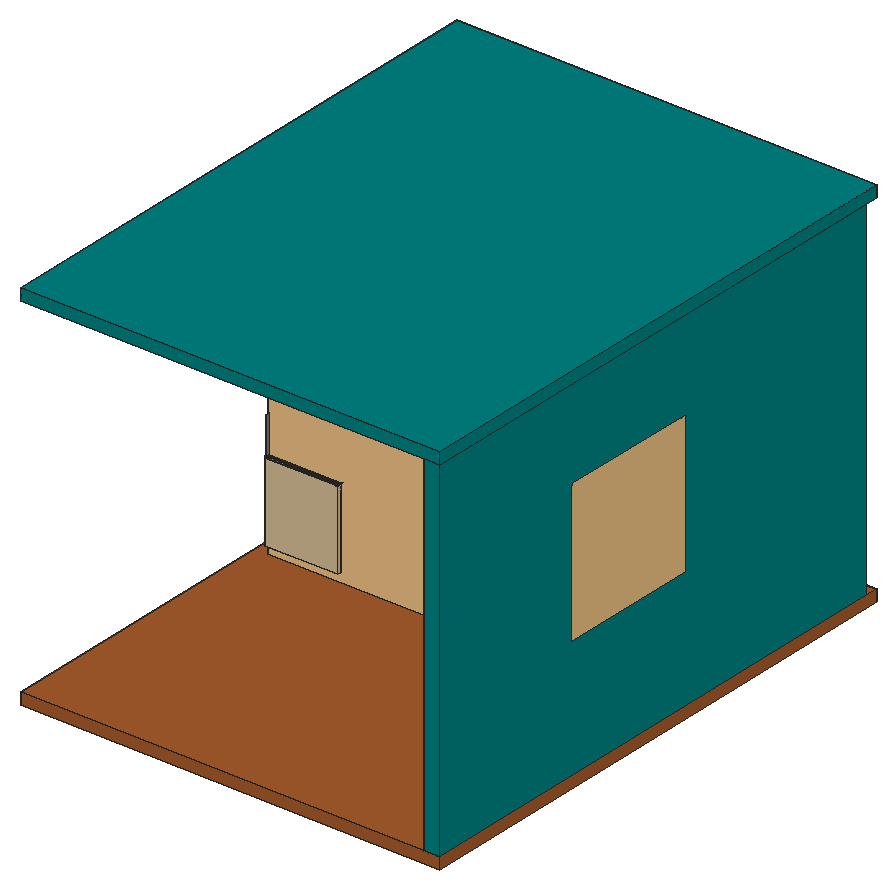
# SketchUp Ruby script. Lengths in inches.
U = 1.inch
M = Sketchup.active_model
def pt(a) = Geom::Point3d.new(a.map { |v| v * U })
def face(e, loops, mat)
  f = e.add_face(loops[0].map { |a| pt(a) })
  loops[1..].each { |l| e.add_face(l.map { |a| pt(a) }).erase! }
  f.material = f.back_material = mat if mat
  f
end
# faces: each face lists its corners as indices into pts; further lists are holes
def faces(e, pts, list, mat = nil) = list.each { |f| face(e, (f[0].is_a?(Array) ? f : [f]).map { |l| l.map { |i| pts[i] } }, mat) }
# xy, xz, yz: faces in a plane at the given z, y or x. An outline is a flat list of corners, or four numbers for a rectangle; further outlines are holes
def ring(l) = l.size == 4 ? [[l[0], l[1]], [l[2], l[1]], [l[2], l[3]], [l[0], l[3]]] : l.each_slice(2).to_a
def flat(e, list, mat, &to3) = list.each { |f| face(e, (f[0].is_a?(Array) ? f : [f]).map { |l| ring(l).map { |u, v| to3.(u, v) } }, mat) }
def xy(e, z, list, mat = nil) = flat(e, list, mat) { |x, y| [x, y, z] }
def xz(e, y, list, mat = nil) = flat(e, list, mat) { |x, z| [x, y, z] }
def yz(e, x, list, mat = nil) = flat(e, list, mat) { |y, z| [x, y, z] }
def lines(e, pts, list) = list.each { |a, b| e.add_line(pt(pts[a]), pt(pts[b])) }
# prism: a flat outline (further loops are holes) pulled along v
def prism(e, loops, v, mat = nil)
  f = face(e, loops, mat); d = Geom::Vector3d.new(v.map { |x| x * U })
  f.pushpull(f.normal.samedirection?(d) ? d.length : -d.length)
end
def box(e, o, s, mat = nil) = prism(e, [[o, [o[0] + s[0], o[1], o[2]], [o[0] + s[0], o[1] + s[1], o[2]], [o[0], o[1] + s[1], o[2]]]], [0, 0, s[2]], mat)
def at(x, y, z, deg = 0) = Geom::Transformation.translation(pt([x, y, z])) * Geom::Transformation.rotation(ORIGIN, Z_AXIS, deg.degrees)
def axes(o, x, y, z) = Geom::Transformation.new([*x, 0, *y, 0, *z, 0, *pt(o).to_a, 1])
def part(name) = M.definitions.add(name)
# library, detail: a bought-in or finely detailed component or shape, given as its bounding box
def library(name, o, s) = part(name).tap { |d| box(d.entities, o, s) }
def detail(e, o, s) = box(e.add_group.entities, o, s)
def put(e, d, t, mat = nil) = e.add_instance(d, t).tap { |i| i.material = mat if mat }
def group(e, t, mat = nil) = e.add_group.tap { |g| g.transformation = t; g.material = mat if mat }.entities
root = M.entities
M.materials.add("CLC2-PC-Blanc INTER").color = [249, 249, 249]
M.materials.add("Material \#1").color = [0, 0, 0]
M.materials.add("Standardmaterial30").color = [86, 86, 86]
M.materials.add("[0031_PapayaWhip]").color = [199, 195, 183]
M.materials.add("[0031_PapayaWhip]1").color = [211, 117, 3]
M.materials.add("[0079_Teal]").color = [0, 128, 128]
M.materials.add("[0091_MintCream]").color = [201, 113, 3]
M.materials.add("[0099_LightSteelBlue]").color = [176, 196, 222]
M.materials.add("[Blacktop Old 01]").color = [132, 136, 139]
M.materials.add("[Blinds Wood White]").color = [138, 137, 139]
M.materials.add("[Encaustic Tile Circular 01]").color = [123, 123, 122]
M.materials.add("[Formica Beige]").color = [211, 187, 149]
M.materials.add("[Ornate Tile 01]").color = [202, 202, 202]
M.materials.add("[Resin Turquoise]").color = [117, 218, 223]
M.materials.add("[Stone Marble]").color = [143, 138, 136]
M.materials.add("[Stone Vein Gray]").color = [166, 165, 165]
M.materials.add("[Terrazzo Light Blue]").color = [196, 214, 227]
M.materials.add("[Tile Hexagon White]").color = [213, 206, 204]
M.materials.add("[Translucent Glass Gray]").color = [128, 128, 128]
M.materials["[Translucent Glass Gray]"].alpha = 0.5
M.materials.add("[Wood Board Cork]").color = [215, 201, 115]
M.materials.add("[Wood Cherry Original]").color = [152, 86, 42]
M.materials.add("[Wood Square Tile 01]").color = [164, 91, 44]
M.materials.add("utensils_wood_2").color = [89, 58, 24]
c1 = library("Group\#12",[-32.31,-359.75,0.0625],[113.14,110.83,100])
c2 = library("Group\#19",[-370.5625,-274.21,5.8125],[90.77,166.34,120.375])
c3 = library("Group\#17",[-278.11,-348.23,5.8],[187.87,187.87,121.65])
c4 = library("Group\#13",[-77.16,-243.45,0.06],[77.78,77.39,334.5])
c5 = library("Group\#11",[5.16,-238.13,0.06],[77.38,77.77,330.87])
c6 = library("Group\#21",[162.6875,-473.8,0.53],[157.34,166.37,329.78])
c7 = library("Group\#14",[-424.81,-54.29,0.29],[386.66,43.55,222.03])
c8 = library("Group\#20",[70.49,-356.56,0.0625],[143.03,166.7,314.72])
c9 = library("Group\#22",[-91.3125,-441.93,-0.01],[120,70.11,138.07])
c10 = library("Group\#16",[-375.96,-353.73,0.05],[297.45,297.44,31.27])
c11 = library("Group\#18",[-284.5,-166.25,5.875],[106.63,106.63,250.48])
c12 = part("Kitchen countertop accessories")
p = [[424.81,473.8,0.01],[425.81,473.8,0.01],[425.81,474.8,0.01]]
lines(c12.entities,p,[[0,1],[2,0]])
put(c12.entities,c1,at(424.81,473.8,0.01))
put(c12.entities,c2,at(424.81,473.8,0.01))
put(c12.entities,c3,at(424.81,473.8,0.01))
put(c12.entities,c4,at(424.81,473.8,0.01))
put(c12.entities,c5,at(424.81,473.8,0.01))
put(c12.entities,c6,at(424.81,473.8,0.01))
put(c12.entities,c7,at(424.81,473.8,0.01),"utensils_wood_2")
put(c12.entities,c8,at(424.81,473.8,0.01))
put(c12.entities,c9,at(424.81,473.8,0.01))
put(c12.entities,c10,at(424.81,473.8,0.01))
put(c12.entities,c11,at(424.81,473.8,0.01))
c13 = library("007",[-28.95,-65.99,21.26],[5.48,1.13,0.69])
c14 = library("Hob1",[-15.52,-17.72,0],[31.04,35.44,3.4])
c15 = library("6-FOUR H60 CLC2",[0,-1.15,0],[23.5,21.54,23.5])
c16 = library("2-TABLE DE CUISSON CLC2",[-11.42,-10.04,0],[22.84,20.08,1.26])
c17 = part("CLC2-Ele02")
prism(c17.entities,[[[0.84,-0.32,0.16],[0.84,-0.33,0.02],[0.84,-0.34,-0.125],[0.84,-0.36,-0.27],[0.84,-0.39,-0.41],[0.84,-0.43,-0.55],[0.84,-0.47,-0.68],[0.84,-0.51,-0.82],[0.84,-0.2,-0.84],[0.84,-0.07,0.84],[0.84,-0.375,0.87],[0.84,-0.35,0.73],[0.84,-0.33,0.59],[0.84,-0.32,0.44],[0.84,-0.32,0.3]]],[-0.83,0,0],"CLC2-PC-Blanc INTER")
prism(c17.entities,[[[-0.01,-0.32,0.16],[-0.01,-0.33,0.02],[-0.01,-0.34,-0.125],[-0.01,-0.36,-0.27],[-0.01,-0.39,-0.41],[-0.01,-0.43,-0.55],[-0.01,-0.47,-0.68],[-0.01,-0.51,-0.82],[-0.01,-0.2,-0.84],[-0.01,-0.07,0.84],[-0.01,-0.375,0.87],[-0.01,-0.35,0.73],[-0.01,-0.33,0.59],[-0.01,-0.32,0.44],[-0.01,-0.32,0.3]]],[-0.83,0,0],"CLC2-PC-Blanc INTER")
xy(c17.entities,-1.57,[[-1.44,-0.19,1.44,0]],"CLC2-PC-Blanc INTER")
xy(c17.entities,-1.5,[[-1.375,-0.12,1.375,0]],"CLC2-PC-Blanc INTER")
xy(c17.entities,-0.87,[[-0.85,-0.29,0.85,-0.12]],"CLC2-PC-Blanc INTER")
xy(c17.entities,0.87,[[-0.85,-0.29,0.85,-0.12]],"CLC2-PC-Blanc INTER")
xy(c17.entities,1.5,[[-1.375,-0.12,1.375,0]],"CLC2-PC-Blanc INTER")
xy(c17.entities,1.57,[[-1.44,-0.19,1.44,0]],"CLC2-PC-Blanc INTER")
xz(c17.entities,-0.12,[[[-1.375,-1.5,-1.41,-1.3,-1.4375,-1.04,-1.46,-0.78,-1.48,-0.52,-1.5,0,-1.48,0.52,-1.46,0.78,-1.4375,1.04,-1.41,1.3,-1.375,1.5,1.375,1.5,1.41,1.3,1.4375,1.04,1.46,0.78,1.48,0.52,1.5,0,1.48,-0.52,1.46,-0.78,1.4375,-1.04,1.41,-1.3,1.375,-1.5],[-0.85,-0.87,0.85,0.87]]],"CLC2-PC-Blanc INTER")
xz(c17.entities,0,[[-1.44,-1.57,-1.48,-1.3125,-1.51,-1.05,-1.54,-0.79,-1.56,-0.53,-1.57,-0.26,-1.57,0.26,-1.56,0.53,-1.54,0.79,-1.51,1.05,-1.48,1.3125,-1.44,1.57,0,1.57,0,1.5,-1.375,1.5,-1.41,1.3,-1.4375,1.04,-1.46,0.78,-1.48,0.52,-1.5,0,-1.48,-0.52,-1.46,-0.78,-1.4375,-1.04,-1.41,-1.3,-1.375,-1.5,0,-1.5,0,-1.57],[0,-1.57,0,-1.5,1.375,-1.5,1.41,-1.3,1.4375,-1.04,1.46,-0.78,1.48,-0.52,1.5,0,1.48,0.52,1.46,0.78,1.4375,1.04,1.41,1.3,1.375,1.5,0,1.5,0,1.57,1.44,1.57,1.48,1.3125,1.51,1.05,1.54,0.79,1.56,0.53,1.57,0.26,1.57,-0.26,1.56,-0.53,1.54,-0.79,1.51,-1.05,1.48,-1.3125,1.44,-1.57]],"CLC2-PC-Blanc INTER")
yz(c17.entities,-1.57,[[-0.0625,-0.26,-0.06,0,0,0,0,-0.26],[-0.06,0,-0.0625,0.26,0,0.26,0,0]],"CLC2-PC-Blanc INTER")
yz(c17.entities,-0.85,[[-0.29,-0.87,-0.12,-0.87,-0.12,0.87,-0.29,0.87,-0.29,0.79,-0.3125,0.53,-0.32,0.26,-0.33,0,-0.32,-0.26,-0.3125,-0.53,-0.29,-0.79]],"CLC2-PC-Blanc INTER")
yz(c17.entities,0.85,[[-0.29,-0.87,-0.29,-0.79,-0.3125,-0.53,-0.32,-0.26,-0.33,0,-0.32,0.26,-0.3125,0.53,-0.29,0.79,-0.29,0.87,-0.12,0.87,-0.12,-0.87]],"CLC2-PC-Blanc INTER")
yz(c17.entities,1.57,[[-0.0625,-0.26,0,-0.26,0,0,-0.06,0],[-0.06,0,0,0,0,0.26,-0.0625,0.26]],"CLC2-PC-Blanc INTER")
p = [[-1.32,-0.3125,0.53],[-1.34,-0.29,0.79],[-1.37,-0.27,1.05],[-1.4,-0.23,1.3125],[-1.44,-0.19,1.57],[-1.48,-0.15,1.3125],
  [-1.51,-0.12,1.05],[-1.54,-0.09,0.79],[-1.56,-0.07,0.53],[-1.57,-0.0625,0.26],[-1.57,-0.06,0],[-1.57,-0.0625,-0.26],
  [-1.56,-0.07,-0.53],[-1.54,-0.09,-0.79],[-1.51,-0.12,-1.05],[-1.48,-0.15,-1.3125],[-1.44,-0.19,-1.57],[-1.4,-0.23,-1.3125],
  [-1.37,-0.27,-1.05],[-1.34,-0.29,-0.79],[-1.32,-0.3125,-0.53],[-1.31,-0.32,-0.26],[-1.3,-0.33,0],[-1.31,-0.32,0.26],
  [1.34,-0.29,0.79],[1.32,-0.3125,0.53],[1.31,-0.32,0.26],[1.3,-0.33,0],[1.31,-0.32,-0.26],[1.32,-0.3125,-0.53],
  [1.34,-0.29,-0.79],[1.37,-0.27,-1.05],[1.4,-0.23,-1.3125],[1.44,-0.19,-1.57],[1.48,-0.15,-1.3125],[1.51,-0.12,-1.05],
  [1.54,-0.09,-0.79],[1.56,-0.07,-0.53],[1.57,-0.0625,-0.26],[1.57,-0.06,0],[1.57,-0.0625,0.26],[1.56,-0.07,0.53],
  [1.54,-0.09,0.79],[1.51,-0.12,1.05],[1.48,-0.15,1.3125],[1.44,-0.19,1.57],[1.4,-0.23,1.3125],[1.37,-0.27,1.05],
  [-1.44,0,-1.57],[-1.48,0,-1.3125],[1.44,0,-1.57],[1.48,0,-1.3125],[-1.375,0,-1.5],[-1.41,0,-1.3],
  [-1.41,-0.12,-1.3],[-1.375,-0.12,-1.5],[1.41,0,-1.3],[1.375,0,-1.5],[1.375,-0.12,-1.5],[1.41,-0.12,-1.3],
  [-1.51,0,-1.05],[1.51,0,-1.05],[-1.4375,0,-1.04],[-1.4375,-0.12,-1.04],[1.4375,0,-1.04],[1.4375,-0.12,-1.04],
  [0.85,-0.29,-0.87],[-0.85,-0.29,-0.87],[-0.85,-0.29,-0.79],[-1.33,-0.29,-0.79],[1.33,-0.29,-0.79],[0.85,-0.29,-0.79],
  [-1.54,0,-0.79],[1.54,0,-0.79],[-1.46,0,-0.78],[-1.46,-0.12,-0.78],[1.46,0,-0.78],[1.46,-0.12,-0.78],
  [-0.85,-0.3125,-0.53],[0.85,-0.3125,-0.53],[-1.56,0,-0.53],[-1.48,0,-0.52],[-1.48,-0.12,-0.52],[1.48,0,-0.52],
  [1.48,-0.12,-0.52],[1.56,0,-0.53],[-0.85,-0.32,-0.26],[0.85,-0.32,-0.26],[-1.57,0,-0.26],[-1.49,0,-0.26],
  [-1.49,-0.12,-0.26],[1.49,0,-0.26],[1.49,-0.12,-0.26],[1.57,0,-0.26],[-0.85,-0.33,0],[0.85,-0.33,0],
  [-1.5,0,0],[-1.5,-0.12,0],[1.5,0,0],[1.5,-0.12,0],[-0.85,-0.32,0.26],[0.85,-0.32,0.26],
  [-1.49,0,0.26],[-1.49,-0.12,0.26],[1.49,0,0.26],[1.49,-0.12,0.26],[-0.85,-0.3125,0.53],[0.85,-0.3125,0.53],
  [-1.57,0,0.26],[-1.56,0,0.53],[-1.48,0,0.52],[-1.48,-0.12,0.52],[1.48,0,0.52],[1.48,-0.12,0.52],
  [1.57,0,0.26],[1.56,0,0.53],[-0.85,-0.29,0.79],[-1.33,-0.29,0.79],[1.33,-0.29,0.79],[0.85,-0.29,0.79],
  [-1.54,0,0.79],[-1.46,0,0.78],[-1.46,-0.12,0.78],[1.46,0,0.78],[1.46,-0.12,0.78],[1.54,0,0.79],
  [-0.85,-0.29,0.87],[0.85,-0.29,0.87],[-1.4375,0,1.04],[-1.4375,-0.12,1.04],[-1.51,0,1.05],[1.4375,0,1.04],
  [1.4375,-0.12,1.04],[1.51,0,1.05],[-1.41,0,1.3],[-1.41,-0.12,1.3],[1.41,0,1.3],[1.41,-0.12,1.3],
  [-1.48,0,1.3125],[1.48,0,1.3125],[-1.44,0,1.57],[1.44,0,1.57],[-1.375,0,1.5],[-1.375,-0.12,1.5],
  [1.375,0,1.5],[1.375,-0.12,1.5]]
faces(c17.entities,p,[[0,1,2,3,4,5,6,7,8,9,10,11,12,13,14,15,16,17,18,19,20,21,22,23],[24,25,26,27,28,29,30,31,32,33,34,35,36,37,38,39,40,41,42,43,44,45,46,47],[48,16,15,49],[32,17,16,33],[33,50,51,34],[52,53,54,55],[56,57,58,59],[31,18,17,32],
  [49,15,14,60],[34,51,61,35],[53,62,63,54],[64,56,59,65],[66,67,68,69,19,18,31,30,70,71],[60,14,13,72],[35,61,73,36],[62,74,75,63],
  [76,64,65,77],[69,68,78,20,19],[71,70,30,29,79],[72,13,12,80],[74,81,82,75],[83,76,77,84],[36,73,85,37],[20,78,86,21],
  [79,29,28,87],[80,12,11,88],[81,89,90,82],[91,83,84,92],[37,85,93,38],[21,86,94,22],[87,28,27,95],[89,96,97,90],
  [98,91,92,99],[22,94,100,23],[95,27,26,101],[96,102,103,97],[104,98,99,105],[23,100,106,0],[101,26,25,107],[108,9,8,109],
  [102,110,111,103],[112,104,105,113],[40,114,115,41],[0,106,116,117,1],[107,25,24,118,119],[109,8,7,120],[110,121,122,111],[123,112,113,124],
  [41,115,125,42],[116,126,127,119,118,24,47,2,1,117],[121,128,129,122],[120,7,6,130],[131,123,124,132],[42,125,133,43],[128,134,135,129],[136,131,132,137],
  [46,3,2,47],[130,6,5,138],[43,133,139,44],[138,5,4,140],[4,3,46,45],[44,139,141,45],[134,142,143,135],[144,136,137,145]],"CLC2-PC-Blanc INTER")
c18 = part("2-PRISEELC CLC2")
put(c18.entities,c17,axes([0,0,0],[1,0,0],[0,0,-1],[0,1,0]))
c19 = library("15-PRODUITS CUISINE CLC2",[-1.94,-2.15,0],[3.93,3.94,5.51])
c20 = library("12-PRODUITS CUISINE CLC2",[-1.08,-1.08,0],[2.16,2.16,5.375])
c21 = library("15-PRODUITS CUISINE CLC2\#1",[-1.94,-2.15,0],[3.93,3.94,5.51])
c22 = library("Sink with drainer",[-0.15,-0.12,-6.4],[37.85,20.23,20.6])
c23 = library("AS-120-mm",[0,0,0],[48,4.72,48])
c24 = library("9-POIGNEE CLC2",[-3.01,-0.26,0],[6.02,0.52,1.49])
c25 = library("2-POIGNEE CLC2",[-2.66,-0.49,0],[5.32,0.98,1.3])
c26 = library("Group\#4",[0,32.625,0],[131,82,57])
c27 = part("Union")
xy(c27.entities,0,[[0,51.67,0.1,82.93]],"[Tile Hexagon White]")
xy(c27.entities,0.04,[[0.1875,0,0,51.67,0.1,51.67,0.29,0]],"[Tile Hexagon White]")
xy(c27.entities,12.44,[[0.1875,0,0.29,0,0.1,51.67,0,51.67]],"[Tile Hexagon White]")
xy(c27.entities,29.375,[[0,51.67,0.1,82.93]],"[Tile Hexagon White]")
xz(c27.entities,0,[[0.1875,0.04,0.29,12.44]],"[Tile Hexagon White]")
xz(c27.entities,51.67,[[0,0,0.1,0.04],[0,12.44,0.1,29.375]],"[Tile Hexagon White]")
xz(c27.entities,82.93,[[0,0,0.1,29.375]],"[Tile Hexagon White]")
yz(c27.entities,0,[[51.67,0,82.93,29.375]],"[Tile Hexagon White]")
yz(c27.entities,0.1,[[51.67,0,82.93,29.375]],"[Encaustic Tile Circular 01]")
p = [[0,51.67,0.04],[0.1875,0,0.04],[0.1875,0,12.44],[0,51.67,12.44],[0.29,0,0.04],[0.1,51.67,0.04],
  [0.1,51.67,12.44],[0.29,0,12.44]]
faces(c27.entities,p,[[0,1,2,3]],"[Tile Hexagon White]")
faces(c27.entities,p,[[4,5,6,7]],"[Encaustic Tile Circular 01]")
c28 = part("Group\#39")
box(c28.entities,[0,-0.16,0],[14.04,0.16,8.44])
c29 = library("Group\#36",[0,0,0],[13.37,2.97,7.55])
c30 = part("Union\#1")
xy(c30.entities,0,[[0,48.27,0.1,124.86]])
xy(c30.entities,0,[[0,0,0.1,48.27]],"[Encaustic Tile Circular 01]")
xy(c30.entities,10.36,[[0,0,0.1,47.52]],"[Encaustic Tile Circular 01]")
xy(c30.entities,29.13,[[0,47.52,0.1,124.86]])
xz(c30.entities,0,[[0,0,0.1,10.36]],"[Encaustic Tile Circular 01]")
xz(c30.entities,47.52,[[0,10.36,0.1,29.13]])
xz(c30.entities,124.86,[[0,0,0.1,29.13]])
yz(c30.entities,0,[[0,0,0,10.36,47.52,10.36,47.52,29.13,124.86,29.13,124.86,0]],"[Encaustic Tile Circular 01]")
yz(c30.entities,0.1,[[48.27,0,124.86,0,124.86,29.13,47.52,29.13,47.52,10.36,48.27,10.36]])
yz(c30.entities,0.1,[[0,0,48.27,10.36]],"[Encaustic Tile Circular 01]")
c31 = library("Group\#182",[0,0,0],[42.16,31.84,40.44])
c32 = library("Group\#184",[0,0,-7.25],[98.84,110.93,7.25])
xz(root,161.23,[[99.375,31.2,126.76,31.21]],"[Stone Vein Gray]")
xz(root,176.99,[[99.375,31.2,126.76,31.21]],"[Stone Vein Gray]")
yz(root,99.375,[[161.23,31.2,176.99,31.21]],"[Stone Vein Gray]")
p = [[29.43,157.1875,3],[29.43,157.1875,30],[126.76,161.23,31.2],[126.76,176.99,31.2],[0,18.6875,120],[0,186.6875,120],
  [143.41,186.6875,120]]
lines(root,p,[[0,1],[2,3],[4,5],[5,6]])
put(root,c12,axes([19.84,158.83,30.625],[0,0.0275,0],[-0.0275,0,0],[0,0,0.0275]))
put(root,c13,axes([77.75,192.75,48.53],[0,0,0.87],[0,0.5481,0],[-0.87,0,0]))
put(root,c13,axes([71.76,192.75,48.53],[0,0,0.87],[0,0.5481,0],[-0.87,0,0]))
put(root,c13,axes([53.76,192.74,48.77],[0,0,0.87],[0,0.5481,0],[-0.87,0,0]))
put(root,c13,axes([95.6,192.75,52.97],[0,0,0.87],[0,0.5481,0],[-0.87,0,0]))
put(root,c13,axes([113.81,192.75,48.53],[0,0,0.87],[0,0.5481,0],[-0.87,0,0]))
put(root,c13,axes([141.37,192.75,48.53],[0,0,0.87],[0,0.5481,0],[-0.87,0,0]))
put(root,c13,axes([143.24,192.75,48.53],[0,0,0.87],[0,0.5481,0],[-0.87,0,0]))
put(root,c13,axes([-6.01,115.6,38.68],[0,-0.87,0],[-0.5481,0,0],[0,0,-0.87]))
put(root,c13,axes([-6.05,129.48,46.95],[0,0,0.87],[-0.5481,0,0],[0,-0.87,0]))
put(root,c13,axes([-6.05,132.24,46.95],[0,0,0.87],[-0.5481,0,0],[0,-0.87,0]))
put(root,c13,axes([-6.05,115.6,44.93],[0,-0.87,0],[-0.5481,0,0],[0,0,-0.87]))
put(root,c13,axes([-5.95,115.6,33.24],[0,-0.87,0],[-0.5481,0,0],[0,0,-0.87]))
put(root,c14,axes([16.75,138.99,30.625],[0.68089,0,0],[0,0.79341,0],[0,0,1.1662]),"Material \#1")
put(root,c15,axes([51.02,159.49,30.625],[1,0,0],[0,1,0],[0,0,1.05]))
put(root,c16,at(16.86,138.26,30.625))
put(root,c18,axes([18.77,181.49,47.7],[1,0,0],[0,0,1],[0,-1,0]))
put(root,c19,axes([75.13,173.46,72.5],[1.17,0,0],[0,1.17,0],[0,0,1.07359]))
put(root,c20,axes([85.96,170.82,72.5],[1.17,0,0],[0,1.17,0],[0,0,1.07359]))
put(root,c21,axes([79.76,173.46,72.5],[1.17,0,0],[0,1.17,0],[0,0,1.07359]))
put(root,c20,axes([83.6,173.46,72.5],[1.17,0,0],[0,1.17,0],[0,0,1.07359]))
put(root,c22,axes([96.12,161.06,31.38],[1,0,0],[0,1,-0.00308],[0,0.00308,1]))
put(root,c23,at(143.41,56.625,41.24,90))
put(root,c24,axes([18.44,167.1875,73.7],[1,0,0],[0,0,0.99928],[0,-1.00073,0]))
put(root,c24,axes([18.44,167.1875,61.05],[1,0,0],[0,0,0.99928],[0,-1.00073,0]))
put(root,c24,axes([122.88,167.1875,73.7],[1,0,0],[0,0,0.99928],[0,-1.00073,0]))
put(root,c24,axes([122.88,167.1875,61.05],[1,0,0],[0,0,0.99928],[0,-1.00073,0]))
put(root,c25,axes([37.15,167.1875,73.34],[0,0,1],[-1,0,0],[0,-1,0]))
put(root,c25,axes([91.29,167.1875,73.34],[0,0,1],[-1,0,0],[0,-1,0]))
put(root,c26,at(4.5,67.5625,0),"[Terrazzo Light Blue]")
g1 = group(root,at(4.5,182.1875,60),"[Wood Board Cork]")
xy(g1,0,[[1,-14,49.09,0],[85.16,-14,133,0]],"[Wood Board Cork]")
xy(g1,11.5,[[49.09,-14,85.16,0]],"[Wood Board Cork]")
xy(g1,12.5,[[50.09,-14,84.16,-0.75]],"[0031_PapayaWhip]")
xy(g1,22.94,[[50.09,-14,84.16,-0.75]],"[0031_PapayaWhip]")
xy(g1,23.94,[[1,-14,49.09,0],[49.09,-14,85.16,0],[85.16,-14,133,0]],"[Wood Board Cork]")
xz(g1,-14,[[1,0,49.09,23.94],[85.16,0,133,23.94],[[49.09,11.5,85.16,23.94],[50.09,12.5,84.16,22.94]]],"[0031_PapayaWhip]")
xz(g1,-0.75,[[50.09,12.5,84.16,22.94]],"[0031_PapayaWhip]")
xz(g1,0,[[1,0,1,23.94,133,23.94,133,0,85.16,0,85.16,11.5,49.09,11.5,49.09,0]],"[0031_PapayaWhip]")
yz(g1,1,[[-14,0,0,23.94]],"[0031_PapayaWhip]")
yz(g1,49.09,[[-14,0,0,11.5]],"[Wood Board Cork]")
yz(g1,84.16,[[-14,12.5,-0.75,22.94]],"[0031_PapayaWhip]")
yz(g1,85.16,[[-14,0,0,11.5]],"[Wood Board Cork]")
yz(g1,133,[[-14,0,0,23.94]],"[0031_PapayaWhip]")
g2 = group(g1,at(50.09,-14,12.5))
yz(g2,0,[[0,0,13.25,10.44]])
g3 = group(root,at(4.5,168.1875,60),"[Blinds Wood White]")
box(g3,[31.16,-1,0],[17.93,1,23.94],"[0031_PapayaWhip]")
xy(g3,0,[[85.16,-1,103,0]],"[0031_PapayaWhip]")
xy(g3,23.94,[[85.16,-1,103,0]],"[0031_PapayaWhip]")
xz(g3,-1,[[85.16,0,103,23.94]],"[0031_PapayaWhip]")
xz(g3,0,[[85.16,0,103,23.94]],"[0031_PapayaWhip]")
yz(g3,85.16,[[-1,0,0,23.94]],"[0031_PapayaWhip]")
yz(g3,103,[[-1,0,0,23.94]],"[0031_PapayaWhip]")
p = [[84,-0.34,22.94],[84,-0.54,22.94]]
lines(g3,p,[[0,1]])
g4 = group(g3,at(0,-1,0),"[Wood Board Cork]")
xy(g4,0,[[0,0,1,15],[1,0,31,1]],"[Wood Board Cork]")
xy(g4,11.89,[[1,0,31,1]],"[Wood Board Cork]")
xy(g4,12.05,[[1,0,31,1]],"[0091_MintCream]")
xy(g4,23.94,[[0,0,1,15],[1,0,31,1]],"[Wood Board Cork]")
xz(g4,0,[[0,0,1,23.94],[1,0,31,11.89],[1,12.05,31,23.94]],"[Wood Board Cork]")
xz(g4,1,[[1,0,31,11.89],[1,11.89,31,12.05],[1,12.05,31,23.94]],"[0091_MintCream]")
xz(g4,15,[[0,0,1,23.94]],"[0091_MintCream]")
yz(g4,0,[[0,0,15,23.94]],"[0091_MintCream]")
yz(g4,1,[[0,0,1,11.89],[1,0,15,23.94],[0,11.89,1,12.05],[0,12.05,1,23.94]],"[0091_MintCream]")
yz(g4,31,[[0,0,1,11.89],[0,12.05,1,23.94]],"[Wood Board Cork]")
g5 = group(g3,at(103.16,-1,12.05),"[Wood Board Cork]")
xy(g5,0,[[0,0,29.84,1]],"[0031_PapayaWhip]1")
xy(g5,11.89,[[0,0,29.84,1]],"[Wood Board Cork]")
xz(g5,0,[[0,0,29.84,11.89]],"[Wood Board Cork]")
xz(g5,1,[[0,0,29.84,11.89]],"[0031_PapayaWhip]1")
yz(g5,0,[[0,0,1,11.89]],"[Wood Board Cork]")
yz(g5,29.84,[[0,0,1,11.89]],"[Wood Board Cork]")
g6 = group(g3,at(103.16,-1,0),"[Wood Board Cork]")
xy(g6,0,[[0,0,29.84,1]],"[Wood Board Cork]")
xy(g6,11.89,[[0,0,29.84,1]],"[Wood Board Cork]")
xz(g6,0,[[0,0,29.84,11.89]],"[Wood Board Cork]")
xz(g6,1,[[0,0,29.84,11.89]],"[Wood Cherry Original]")
yz(g6,0,[[0,0,1,11.89]],"[Wood Cherry Original]")
yz(g6,29.84,[[0,0,1,11.89]],"[Wood Board Cork]")
g7 = group(g3,at(133.16,-1,0),"[Wood Board Cork]")
xy(g7,0,[[0,0,2.25,15]],"[Wood Board Cork]")
xy(g7,23.94,[[0,0,2.25,15]],"[Wood Board Cork]")
xz(g7,0,[[0,0,2.25,23.94]],"[Wood Board Cork]")
xz(g7,15,[[0,0,2.25,23.94]],"[Wood Cherry Original]")
yz(g7,0,[[0,0,1,23.94],[1,0,15,23.94]],"[Wood Cherry Original]")
yz(g7,2.25,[[0,0,15,23.94]],"[Wood Board Cork]")
g8 = group(root,at(54.59,168.1875,72.5))
box(g8,[-1,0,0],[1,13.25,10.44])
g9 = group(root,at(28.5,67.5625,3),"[Formica Beige]")
box(g9,[0,56.625,0],[1,29.84,13.54])
box(g9,[0,56.625,20.35],[1,29.84,6.65])
box(g9,[0,56.625,13.62],[1,29.84,6.65])
xy(g9,0,[[0,32.625,1,44.42],[0,44.58,1,56.47]])
xy(g9,0,[[-24,31.5,1,32.47]],"[Terrazzo Light Blue]")
xy(g9,26.1,[[0.125,32.72,1,44.32],[0.125,44.68,1,56.37]],"Standardmaterial30")
xy(g9,26.78,[[0.5625,32.72,1,44.32],[0.57,44.68,1,56.37]],"Standardmaterial30")
xy(g9,26.9,[[0.125,32.72,0.5625,44.32],[0.125,44.68,0.57,56.37]])
xy(g9,27,[[0,32.625,1,44.42],[0,44.58,1,56.47]])
xy(g9,27,[[-24,31.5,1,32.47]],"[Terrazzo Light Blue]")
xz(g9,31.5,[[-24,0,1,27]],"[Formica Beige]")
xz(g9,32.47,[[-24,0,1,27]],"[Terrazzo Light Blue]")
xz(g9,32.625,[[0,0,1,27]])
xz(g9,32.72,[[0.125,26.1,0.125,26.9,0.5625,26.9,0.5625,26.78,1,26.78,1,26.1]],"Standardmaterial30")
xz(g9,44.32,[[0.125,26.1,1,26.1,1,26.78,0.5625,26.78,0.5625,26.9,0.125,26.9]],"Standardmaterial30")
xz(g9,44.42,[[0,0,1,27]])
xz(g9,44.58,[[0,0,1,27]])
xz(g9,44.68,[[0.125,26.1,0.125,26.9,0.57,26.9,0.57,26.78,1,26.78,1,26.1]],"Standardmaterial30")
xz(g9,56.37,[[0.125,26.1,1,26.1,1,26.78,0.57,26.78,0.57,26.9,0.125,26.9]],"Standardmaterial30")
xz(g9,56.47,[[0,0,1,27]])
yz(g9,-24,[[31.5,0,32.47,27]],"[Terrazzo Light Blue]")
yz(g9,0,[[32.625,0,44.42,27],[44.42,0,44.58,27],[44.58,0,56.47,27]])
yz(g9,0.125,[[32.72,26.1,44.32,26.9],[44.68,26.1,56.37,26.9]],"Standardmaterial30")
yz(g9,0.5625,[[32.72,26.78,44.32,26.9]])
yz(g9,0.57,[[44.68,26.78,56.37,26.9]])
yz(g9,1,[[[32.625,26,44.42,27],[32.72,26.1,44.32,26.78]],[[44.58,26,56.47,27],[44.68,26.1,56.37,26.78]]])
yz(g9,1,[[31.5,0,32.47,27],[32.625,0,44.42,26],[44.58,0,56.47,26]],"[Formica Beige]")
g10 = group(g9,at(0,86.625,0))
prism(g10,[[[1,3,0],[1,0,0],[0,0,0],[0,4,0],[1,4,0]]],[0,0,27])
g11 = group(root,at(29.5,157.1875,3),"[Stone Marble]")
xy(g11,0,[[22.16,0,28,1],[28.16,0,46,1],[64.16,0,82,1],[82.16,0,94,1],[94.16,0,106,1],
  [106.16,0,108.22,25]])
xy(g11,0,[[4.16,0,22,1]],"[Terrazzo Light Blue]")
xy(g11,27,[[22.16,0,28,1],[28.16,0,46,1],[64.16,0,82,1],[82.16,0,94,1],[94.16,0,106,1]])
xy(g11,27,[[4.16,0,22,1],[106.16,0,108.22,25]],"[Terrazzo Light Blue]")
xz(g11,0,[[4.16,0,22,27],[22.16,0,28,27],[28.16,0,46,27],[64.16,0,82,27],[82.16,0,94,27],
  [94.16,0,106,27],[106.16,0,108.22,27]],"[Formica Beige]")
xz(g11,1,[[22.16,0,28,27],[28.16,0,46,27],[64.16,0,82,27],[82.16,0,94,27],[94.16,0,106,27]])
xz(g11,1,[[4.16,0,22,27]],"[Terrazzo Light Blue]")
xz(g11,25,[[106.16,0,108.22,27]])
yz(g11,4.16,[[0,0,1,27]],"[Terrazzo Light Blue]")
yz(g11,22,[[0,0,1,27]],"[Terrazzo Light Blue]")
yz(g11,22.16,[[0,0,1,27]])
yz(g11,28,[[0,0,1,27]])
yz(g11,28.16,[[0,0,1,27]])
yz(g11,46,[[0,0,1,27]])
yz(g11,64.16,[[0,0,1,27]])
yz(g11,82,[[0,0,1,27]])
yz(g11,82.16,[[0,0,1,27]])
yz(g11,94,[[0,0,1,27]])
yz(g11,94.16,[[0,0,1,27]])
yz(g11,106,[[0,0,1,27]])
yz(g11,106.16,[[0,0,1,27],[1,0,25,27]])
yz(g11,108.22,[[0,0,25,27]],"[Formica Beige]")
g12 = group(g11,at(0,0,0),"[Formica Beige]")
box(g12,[0,0,0],[4,1,27])
g13 = group(root,at(75.5,158.1875,3),"[Formica Beige]")
prism(g13,[[[18.16,0,53.0625],[18.16,0,27],[18.16,0,0],[0,0,0],[0,0,27],[0,0,53.0625]]],[0,-1,0])
g14 = group(root,at(4.5,100.1875,30))
xy(g14,-0.22,[[0,-0.76,0,-0.72,24.6,-0.72,24.64,-0.76],[24.64,-0.76,24.6,-0.72,24.6,57.4,24.64,57.36],[0,-0.72,0,82,71,82,71,57.4,24.6,57.4,24.6,-0.72],[24.64,57.36,24.6,57.4,71,57.4,71,57.36]],"[Stone Vein Gray]")
xy(g14,0.625,[[0,-0.83,24.71,-0.83,24.67,-0.79,0,-0.79],[24.71,-0.83,24.71,57.29,24.67,57.33,24.67,-0.79],[0,-0.79,24.67,-0.79,24.67,57.33,71,57.33,71,82,0,82],[24.71,57.29,71,57.29,71,57.33,24.67,57.33]],"[Stone Vein Gray]")
xz(g14,-1.125,[[0,0,25,0.39]],"[Stone Vein Gray]")
xz(g14,57,[[25,0,71,0.39]],"[Stone Vein Gray]")
xz(g14,82,[[0,-0.22,71,0.625]],"[Stone Vein Gray]")
yz(g14,0,[[-0.76,-0.22,-0.92,-0.18,-0.95,-0.16,-0.99,-0.14,-1.02,-0.12,-1.05,-0.09,-1.08,-0.0625,-1.1,-0.03,-1.125,0,-1.125,0.39,-1.11,0.42,-1.05,0.51,-1,0.56,-0.97,0.58,-0.93,0.6,-0.87,0.62,-0.83,0.625,82,0.625,82,-0.22]],"[Stone Vein Gray]")
yz(g14,25,[[-1.125,0,57,0.39]],"[Stone Vein Gray]")
yz(g14,71,[[57.36,-0.22,82,-0.22,82,0.625,57.29,0.625,57.26,0.62,57.22,0.61,57.19,0.6,57.1,0.54,57.07,0.51,57.01,0.42,57,0.39,57,0,57.02,-0.03,57.05,-0.0625,57.08,-0.09,57.11,-0.12,57.17,-0.16,57.21,-0.18,57.24,-0.19]],"[Stone Vein Gray]")
p = [[0,-0.95,-0.16],[0,-0.92,-0.18],[24.79,-0.92,-0.18],[24.83,-0.95,-0.16],[0,-0.99,-0.14],[24.86,-0.99,-0.14],
  [24.79,57.21,-0.18],[24.83,57.17,-0.16],[24.86,57.14,-0.14],[0,-0.88,-0.19],[0,-0.84,-0.2],[24.72,-0.84,-0.2],
  [24.76,-0.88,-0.19],[24.72,57.28,-0.2],[24.76,57.24,-0.19],[0,-0.8,-0.21],[0,-0.76,-0.22],[24.64,-0.76,-0.22],
  [24.68,-0.8,-0.21],[24.64,57.36,-0.22],[24.68,57.32,-0.21],[71,57.17,-0.16],[71,57.14,-0.14],[71,57.28,-0.2],
  [71,57.24,-0.19],[71,57.21,-0.18],[71,57.36,-0.22],[71,57.32,-0.21],[0,-1.08,-0.0625],[0,-1.05,-0.09],
  [24.92,-1.05,-0.09],[24.95,-1.08,-0.0625],[0,-1.1,-0.03],[24.98,-1.1,-0.03],[24.92,57.08,-0.09],[24.95,57.05,-0.0625],
  [24.98,57.02,-0.03],[0,-1.02,-0.12],[24.89,-1.02,-0.12],[24.89,57.11,-0.12],[71,57.08,-0.09],[71,57.05,-0.0625],
  [71,57.02,-0.03],[71,57.11,-0.12],[0,-1.125,0],[25,-1.125,0],[25,57,0],[71,57,0],
  [0,-1.11,0.42],[0,-1.125,0.39],[25,-1.125,0.39],[24.99,-1.11,0.42],[0,-1.09,0.45],[24.97,-1.09,0.45],
  [25,57,0.39],[24.99,57.01,0.42],[24.97,57.03,0.45],[71,57,0.39],[71,57.01,0.42],[71,57.03,0.45],
  [0,-1.07,0.48],[24.95,-1.07,0.48],[0,-1.05,0.51],[24.93,-1.05,0.51],[0,-1.02,0.54],[24.9,-1.02,0.54],
  [24.95,57.05,0.48],[24.93,57.07,0.51],[24.9,57.1,0.54],[0,-1,0.56],[24.87,-1,0.56],[24.87,57.13,0.56],
  [71,57.05,0.48],[71,57.07,0.51],[71,57.1,0.54],[71,57.13,0.56],[0,-0.97,0.58],[24.84,-0.97,0.58],
  [0,-0.93,0.6],[24.81,-0.93,0.6],[24.84,57.16,0.58],[24.81,57.19,0.6],[0,-0.9,0.61],[24.78,-0.9,0.61],
  [0,-0.87,0.62],[24.74,-0.87,0.62],[0,-0.83,0.625],[24.71,-0.83,0.625],[24.78,57.22,0.61],[24.74,57.26,0.62],
  [24.71,57.29,0.625],[71,57.16,0.58],[71,57.22,0.61],[71,57.26,0.62],[71,57.19,0.6],[71,57.29,0.625],
  [71,82,0],[89.16,82,0],[89.16,58,0]]
faces(g14,p,[[0,1,2,3],[4,0,3,5],[3,2,6,7],[5,3,7,8],[9,10,11,12],[1,9,12,2],[12,11,13,14],[2,12,14,6],
  [15,16,17,18],[10,15,18,11],[18,17,19,20],[11,18,20,13],[8,7,21,22],[14,13,23,24],[6,14,24,25],[7,6,25,21],
  [20,19,26,27],[13,20,27,23],[28,29,30,31],[32,28,31,33],[31,30,34,35],[33,31,35,36],[37,4,5,38],[29,37,38,30],
  [38,5,8,39],[30,38,39,34],[35,34,40,41],[36,35,41,42],[39,8,22,43],[34,39,43,40],[44,32,33,45],[45,33,36,46],
  [46,36,42,47],[48,49,50,51],[52,48,51,53],[51,50,54,55],[53,51,55,56],[55,54,57,58],[56,55,58,59],[60,52,53,61],
  [62,60,61,63],[64,62,63,65],[61,53,56,66],[63,61,66,67],[65,63,67,68],[69,64,65,70],[70,65,68,71],[66,56,59,72],
  [67,66,72,73],[68,67,73,74],[71,68,74,75],[76,69,70,77],[78,76,77,79],[77,70,71,80],[79,77,80,81],[82,78,79,83],
  [84,82,83,85],[86,84,85,87],[85,83,88,89],[87,85,89,90],[83,79,81,88],[80,71,75,91],[89,88,92,93],[81,80,91,94],
  [88,81,94,92],[90,89,93,95]],"[Stone Vein Gray]")
lines(g14,p,[[96,97],[98,97]])
put(root,c27,at(4.5,99.25,30.625))
g15 = group(root,at(0,-53.3125,-4))
box(g15,[0,53.3125,0],[143.41,186.6875,4],"[Wood Square Tile 01]")
g16 = group(root,at(70.84,168.1875,72.5))
box(g16,[0,0,0],[1,13.25,10.44],"[0031_PapayaWhip]")
g17 = group(root,at(71.7,167.1875,71.5))
put(g17,c28,at(1.92,0.66,2),"[Translucent Glass Gray]")
g18 = group(g17,at(0,0,0))
prism(g18,[[[17.96,0,12.44],[0,0,12.44],[0,0,0],[17.96,0,0]],[[15.96,0,10.44],[15.96,0,2],[1.92,0,2],[1.92,0,10.44]]],[0,1,0],"[0099_LightSteelBlue]")
g19 = group(root,at(53.59,167.1875,71.5))
put(g19,c28,at(2,0.66,2),"[Translucent Glass Gray]")
g20 = group(g19,at(0,0,0))
prism(g20,[[[0,1,12.44],[17.96,1,12.44],[17.96,1,0],[0,1,0]],[[16.04,1,2],[16.04,1,10.44],[2,1,10.44],[2,1,2]]],[0,-1,0],"[0099_LightSteelBlue]")
put(root,c29,at(55.46,170.78,72.5))
g21 = group(root,at(138.15,18.6875,0))
prism(g21,[[[0,163.5,0],[0,-18.6875,0],[0,-18.6875,120],[0,163.5,120]],[[0,37.9375,89.24],[0,37.9375,41.24],[0,85.9375,41.24],[0,85.9375,89.24]]],[5.25,0,0],"[0079_Teal]")
g22 = group(root,at(4.5,181.49,30.625),"[Ornate Tile 01]")
box(g22,[132.01,0,0],[1.21,0.7,29.375],"[Ornate Tile 01]")
g23 = group(g22,at(0,0,0),"[Encaustic Tile Circular 01]")
xz(g23,0,[[0,0,132.01,0,132.01,29.375,85.16,29.375,85.16,40.875,49.09,40.875,49.09,29.375,0,29.375]],"[Encaustic Tile Circular 01]")
g24 = group(root,at(4.5,157.1875,23.8125))
xy(g24,0,[[95.806,5.648,109.376,5.685,109.764,5.693,110.148,5.75,110.522,5.854,110.88,6.005,111.216,6.199,111.525,6.435,111.802,6.707,112.043,7.012,112.243,7.345,112.4,7.7,112.51,8.072,112.573,8.456,112.543,18.498,112.519,18.876,112.449,19.248,112.336,19.61,112.18,19.955,111.984,20.279,111.75,20.577,111.482,20.845,111.184,21.079,110.86,21.275,110.515,21.431,110.153,21.544,109.781,21.614,95.609,21.565,95.256,21.526,94.911,21.444,94.579,21.32,94.264,21.157,93.973,20.955,93.708,20.72,93.474,20.453,93.275,20.16,93.113,19.845,92.991,19.512,92.912,19.166,92.875,18.814,92.907,8.379,92.951,8.016,93.04,7.661,93.173,7.321,93.348,7,93.5625,6.703,93.812,6.436,94.094,6.203,94.402,6.007,94.733,5.851,95.081,5.738,95.441,5.67]],"[Stone Vein Gray]")
xy(g24,6.259,[[132.157,0,133.219,25]],"[Stone Vein Gray]")
xy(g24,6.813,[[0,24.3,132.011,25.3125]],"[Tile Hexagon White]")
xy(g24,7.041,[[133.219,0,133.22,25]],"[Stone Vein Gray]")
xy(g24,7.1875,[[[89.157,0.146,133.074,24.3],[95.806,5.648,95.441,5.67,95.081,5.738,94.733,5.851,94.402,6.007,94.094,6.203,93.812,6.436,93.5625,6.703,93.348,7,93.173,7.321,93.04,7.661,92.951,8.016,92.907,8.379,92.875,18.814,92.912,19.166,92.991,19.512,93.113,19.845,93.275,20.16,93.474,20.453,93.708,20.72,93.973,20.955,94.264,21.157,94.579,21.32,94.911,21.444,95.256,21.526,95.609,21.565,109.781,21.614,110.153,21.544,110.515,21.431,110.86,21.275,111.184,21.079,111.482,20.845,111.75,20.577,111.984,20.279,112.18,19.955,112.336,19.61,112.449,19.248,112.519,18.876,112.543,18.498,112.573,8.456,112.51,8.072,112.4,7.7,112.243,7.345,112.043,7.012,111.802,6.707,111.525,6.435,111.216,6.199,110.88,6.005,110.522,5.854,110.148,5.75,109.764,5.693,109.376,5.685]],[89.157,24.3,132.011,25],[132.011,24.3,133.074,25]],"[Stone Vein Gray]")
xy(g24,36.1875,[[0,24.3,49,25.3125],[49,24.3,49.085,25.3125],[85.157,24.3,132.011,25.3125],[49.085,25,85.157,25.3125]],"[Tile Hexagon White]")
xy(g24,47.6875,[[49.085,24.3,85.157,25]],"[Tile Hexagon White]")
xz(g24,0,[[89.157,6.259,133.219,7.041]],"[Stone Vein Gray]")
xz(g24,25,[[132.072,6.181,132.059,6.183,132.047,6.1875,132.047,7.149,132.11,7.149,132.11,6.187,132.098,6.183,132.085,6.181],[132.11,6.187,132.11,7.149,132.011,7.149,132.011,7.1875,133.074,7.1875,133.093,7.186,133.112,7.183,133.13,7.176,133.147,7.168,133.163,7.157,133.177,7.145,133.19,7.13,133.2,7.114,133.209,7.097,133.215,7.079,133.219,7.06,133.22,7.041,133.219,7.041,133.219,6.259,132.157,6.259,132.156,6.246,132.153,6.234,132.148,6.222,132.141,6.211,132.132,6.201,132.122,6.193],[89.157,7.149,132.011,7.1875]],"[Stone Vein Gray]")
xz(g24,25,[[49.085,36.1875,85.157,47.6875]],"[Tile Hexagon White]")
xz(g24,25.3125,[[0,6.813,132.011,36.1875]],"[Tile Hexagon White]")
yz(g24,0,[[24.3,6.813,25.3125,36.1875]],"[Tile Hexagon White]")
yz(g24,49.085,[[24.3,36.1875,25,47.6875]],"[Tile Hexagon White]")
yz(g24,85.157,[[24.3,36.1875,25,47.6875]],"[Tile Hexagon White]")
yz(g24,89.157,[[0.047,6.187,0,6.1875,0,6.259,0.001,6.246,0.004,6.234,0.01,6.222,0.017,6.211,0.026,6.201,0.036,6.193],[0.047,6.187,0.036,6.193,0.026,6.201,0.017,6.211,0.01,6.222,0.004,6.234,0.001,6.246,0,6.259,0,7.041,0.001,7.06,0.005,7.079,0.011,7.097,0.02,7.114,0.03,7.13,0.043,7.145,0.047,7.149,0.057,7.157,0.073,7.168,0.09,7.176,0.108,7.183,0.127,7.186,0.146,7.1875,25,7.1875,25,7.149,0.047,7.149]],"[Stone Vein Gray]")
yz(g24,132.011,[[25,6.813,25.3125,36.1875]],"[Tile Hexagon White]")
yz(g24,132.11,[[0.047,6.187,25,7.149]],"[Stone Vein Gray]")
yz(g24,133.219,[[0,6.259,25,7.041]],"[Stone Vein Gray]")
p = [[95.441,5.67,7.1875],[95.806,5.648,7.1875],[95.806,5.648,0],[95.441,5.67,0],[109.376,5.685,7.1875],[109.376,5.685,0],
  [94.733,5.851,7.1875],[95.081,5.738,7.1875],[95.081,5.738,0],[94.733,5.851,0],[109.764,5.693,7.1875],[109.764,5.693,0],
  [110.148,5.75,7.1875],[110.148,5.75,0],[110.522,5.854,7.1875],[110.522,5.854,0],[94.402,6.007,7.1875],[94.402,6.007,0],
  [110.88,6.005,7.1875],[110.88,6.005,0],[94.094,6.203,7.1875],[94.094,6.203,0],[111.216,6.199,7.1875],[111.216,6.199,0],
  [93.812,6.436,7.1875],[93.812,6.436,0],[111.525,6.435,7.1875],[111.525,6.435,0],[93.5625,6.703,7.1875],[93.5625,6.703,0],
  [111.802,6.707,7.1875],[111.802,6.707,0],[93.348,7,7.1875],[93.348,7,0],[112.043,7.012,7.1875],[112.043,7.012,0],
  [93.173,7.321,7.1875],[93.173,7.321,0],[112.243,7.345,7.1875],[112.243,7.345,0],[93.04,7.661,7.1875],[93.04,7.661,0],
  [112.4,7.7,7.1875],[112.4,7.7,0],[92.951,8.016,7.1875],[92.951,8.016,0],[112.51,8.072,7.1875],[112.51,8.072,0],
  [92.907,8.379,7.1875],[92.907,8.379,0],[112.573,8.456,7.1875],[112.573,8.456,0],[92.875,18.814,7.1875],[92.875,18.814,0],
  [112.543,18.498,7.1875],[112.543,18.498,0],[112.519,18.876,7.1875],[112.519,18.876,0],[92.912,19.166,7.1875],[92.912,19.166,0],
  [112.449,19.248,7.1875],[112.449,19.248,0],[92.991,19.512,7.1875],[92.991,19.512,0],[112.336,19.61,7.1875],[112.336,19.61,0],
  [93.113,19.845,7.1875],[93.113,19.845,0],[112.18,19.955,7.1875],[112.18,19.955,0],[93.275,20.16,7.1875],[93.275,20.16,0],
  [111.984,20.279,7.1875],[111.984,20.279,0],[93.474,20.453,7.1875],[93.474,20.453,0],[111.75,20.577,7.1875],[111.75,20.577,0],
  [93.708,20.72,7.1875],[93.708,20.72,0],[111.482,20.845,7.1875],[111.482,20.845,0],[93.973,20.955,7.1875],[93.973,20.955,0],
  [111.184,21.079,7.1875],[111.184,21.079,0],[94.264,21.157,7.1875],[94.264,21.157,0],[110.86,21.275,7.1875],[110.86,21.275,0],
  [94.579,21.32,7.1875],[94.579,21.32,0],[94.911,21.444,7.1875],[94.911,21.444,0],[110.515,21.431,7.1875],[110.515,21.431,0],
  [95.256,21.526,7.1875],[95.256,21.526,0],[110.153,21.544,7.1875],[110.153,21.544,0],[95.609,21.565,7.1875],[95.609,21.565,0],
  [109.781,21.614,7.1875],[109.781,21.614,0],[132.156,0.001,6.246],[132.157,0,6.259],[89.157,0,6.259],[89.157,0.001,6.246],
  [132.148,0.01,6.222],[132.153,0.004,6.234],[89.157,0.004,6.234],[89.157,0.01,6.222],[132.141,0.017,6.211],[89.157,0.017,6.211],
  [132.122,0.036,6.193],[132.132,0.026,6.201],[89.157,0.026,6.201],[89.157,0.036,6.193],[132.11,0.047,6.187],[89.157,0.047,6.187],
  [132.157,0,6.1875],[89.157,0,6.1875],[132.132,25,6.201],[132.141,25,6.211],[132.157,25,6.1875],[132.11,25,6.187],
  [132.122,25,6.193],[132.148,25,6.222],[132.153,25,6.234],[132.156,25,6.246],[132.157,25,6.259],[133.22,0,7.041],
  [133.219,0.001,7.06],[89.157,0.001,7.06],[89.157,0,7.041],[133.219,0,7.041],[133.22,25,7.041],[133.219,25,7.06],
  [133.19,0.03,7.13],[133.177,0.043,7.145],[89.157,0.043,7.145],[89.157,0.03,7.13],[133.209,0.011,7.097],[133.2,0.02,7.114],
  [89.157,0.02,7.114],[89.157,0.011,7.097],[133.215,0.005,7.079],[89.157,0.005,7.079],[133.163,0.057,7.157],[89.157,0.057,7.157],
  [89.157,0.047,7.149],[133.215,25,7.079],[133.209,25,7.097],[133.2,25,7.114],[133.177,25,7.145],[133.163,25,7.157],
  [133.19,25,7.13],[133.112,0.108,7.183],[133.093,0.127,7.186],[89.157,0.127,7.186],[89.157,0.108,7.183],[133.074,0.146,7.1875],
  [89.157,0.146,7.1875],[133.147,0.073,7.168],[89.157,0.073,7.168],[133.13,0.09,7.176],[89.157,0.09,7.176],[133.093,25,7.186],
  [133.074,25,7.1875],[133.074,24.3,7.1875],[133.13,25,7.176],[133.112,25,7.183],[133.147,25,7.168],[85.157,11,36.1875],
  [85.157,24.3,36.1875],[49,11,36.1875],[49,24.3,36.1875]]
faces(g24,p,[[0,1,2,3],[1,4,5,2],[6,7,8,9],[7,0,3,8],[4,10,11,5],[10,12,13,11],[12,14,15,13],[16,6,9,17],
  [14,18,19,15],[20,16,17,21],[18,22,23,19],[24,20,21,25],[22,26,27,23],[28,24,25,29],[26,30,31,27],[32,28,29,33],
  [30,34,35,31],[36,32,33,37],[34,38,39,35],[40,36,37,41],[38,42,43,39],[44,40,41,45],[42,46,47,43],[48,44,45,49],
  [46,50,51,47],[52,48,49,53],[50,54,55,51],[54,56,57,55],[58,52,53,59],[56,60,61,57],[62,58,59,63],[60,64,65,61],
  [66,62,63,67],[64,68,69,65],[70,66,67,71],[68,72,73,69],[74,70,71,75],[72,76,77,73],[78,74,75,79],[76,80,81,77],
  [82,78,79,83],[80,84,85,81],[86,82,83,87],[84,88,89,85],[90,86,87,91],[92,90,91,93],[88,94,95,89],[96,92,93,97],
  [94,98,99,95],[100,96,97,101],[98,102,103,99],[102,100,101,103],[104,105,106,107],[108,109,110,111],[112,108,111,113],[114,115,116,117],
  [118,114,117,119],[109,104,107,110],[115,112,113,116],[120,118,119,121],[122,123,112,115],[124,125,118,120],[125,126,114,118],[126,122,115,114],
  [123,127,108,112],[127,128,109,108],[129,130,105,104],[128,129,104,109],[131,132,133,134,135],[136,137,132,131],[138,139,140,141],[142,143,144,145],
  [146,142,145,147],[143,138,141,144],[139,148,149,150,140],[132,146,147,133],[137,151,146,132],[151,152,142,146],[152,153,143,142],[154,155,148,139],
  [156,154,139,138],[153,156,138,143],[157,158,159,160],[158,161,162,159],[148,163,164,149],[165,157,160,166],[163,165,166,164],[167,168,169,161,158],
  [170,171,157,165],[172,170,165,163],[171,167,158,157],[155,172,163,148]],"[Stone Vein Gray]")
lines(g24,p,[[173,174],[175,176]])
g25 = group(root,at(0,18.6875,120))
box(g25,[0,-18.6875,0],[143.41,186.6875,4],"[0079_Teal]")
put(root,c30,at(137.72,56.625,30.87))
put(root,c31,at(96,67.54,0))
put(root,c32,at(21.07,44.5,120),"[Resin Turquoise]")
g26 = group(root,at(4,22.6875,120))
xy(g26,-4,[[[0,0,135.41,160],[14.19,19.94,117.4,134.87]]],"[Blacktop Old 01]")
xy(g26,-2.0625,[[14.19,19.94,17.07,132.75],[17.07,19.94,115.9,21.82],[115.9,19.94,117.4,134.87],[14.19,132.75,115.9,134.87]],"[Blacktop Old 01]")
xy(g26,0,[[[0,0,135.41,160],[17.07,21.82,115.9,132.75]]],"[Blacktop Old 01]")
xz(g26,0,[[0,-4,135.41,0]],"[Blacktop Old 01]")
xz(g26,19.94,[[14.19,-4,117.4,-2.0625]],"[Blacktop Old 01]")
xz(g26,21.82,[[17.07,-2.0625,115.9,0]],"[Blacktop Old 01]")
xz(g26,132.75,[[17.07,-2.0625,115.9,0]],"[Blacktop Old 01]")
xz(g26,134.87,[[14.19,-4,117.4,-2.0625]],"[Blacktop Old 01]")
xz(g26,160,[[0,-4,135.41,0]],"[Blacktop Old 01]")
yz(g26,0,[[0,-4,160,0]],"[Blacktop Old 01]")
yz(g26,14.19,[[19.94,-4,134.87,-2.0625]],"[Blacktop Old 01]")
yz(g26,17.07,[[21.82,-2.0625,132.75,0]],"[Blacktop Old 01]")
yz(g26,115.9,[[21.82,-2.0625,132.75,0]],"[Blacktop Old 01]")
yz(g26,117.4,[[19.94,-4,134.87,-2.0625]],"[Blacktop Old 01]")
yz(g26,135.41,[[0,-4,160,0]],"[Blacktop Old 01]")
p = [[134.15,0,0],[134.15,159.5,0]]
lines(g26,p,[[0,1]])
